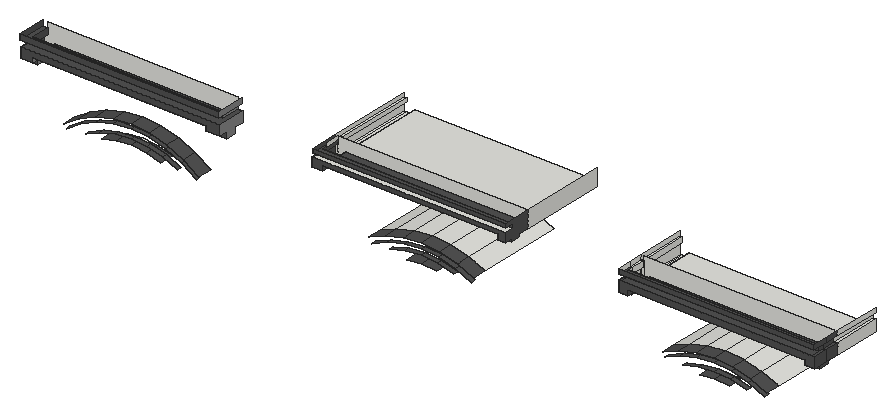
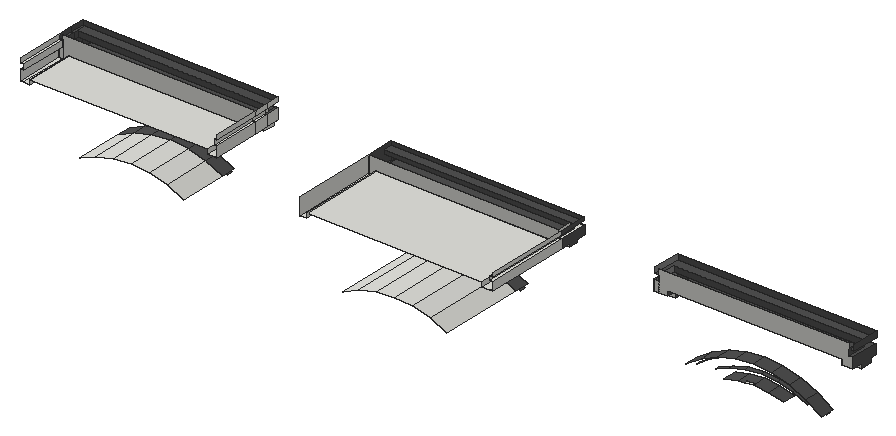
# SketchUp Ruby script. Lengths in inches.
U = 1.inch
M = Sketchup.active_model
def pt(a) = Geom::Point3d.new(a.map { |v| v * U })
def face(e, loops, mat)
  f = e.add_face(loops[0].map { |a| pt(a) })
  loops[1..].each { |l| e.add_face(l.map { |a| pt(a) }).erase! }
  f.material = f.back_material = mat if mat
  f
end
# faces: each face lists its corners as indices into pts; further lists are holes
def faces(e, pts, list, mat = nil) = list.each { |f| face(e, (f[0].is_a?(Array) ? f : [f]).map { |l| l.map { |i| pts[i] } }, mat) }
# xy, xz, yz: faces in a plane at the given z, y or x. An outline is a flat list of corners, or four numbers for a rectangle; further outlines are holes
def ring(l) = l.size == 4 ? [[l[0], l[1]], [l[2], l[1]], [l[2], l[3]], [l[0], l[3]]] : l.each_slice(2).to_a
def flat(e, list, mat, &to3) = list.each { |f| face(e, (f[0].is_a?(Array) ? f : [f]).map { |l| ring(l).map { |u, v| to3.(u, v) } }, mat) }
def xy(e, z, list, mat = nil) = flat(e, list, mat) { |x, y| [x, y, z] }
def xz(e, y, list, mat = nil) = flat(e, list, mat) { |x, z| [x, y, z] }
def yz(e, x, list, mat = nil) = flat(e, list, mat) { |y, z| [x, y, z] }
def lines(e, pts, list) = list.each { |a, b| e.add_line(pt(pts[a]), pt(pts[b])) }
# prism: a flat outline (further loops are holes) pulled along v
def prism(e, loops, v, mat = nil)
  f = face(e, loops, mat); d = Geom::Vector3d.new(v.map { |x| x * U })
  f.pushpull(f.normal.samedirection?(d) ? d.length : -d.length)
end
def box(e, o, s, mat = nil) = prism(e, [[o, [o[0] + s[0], o[1], o[2]], [o[0] + s[0], o[1] + s[1], o[2]], [o[0], o[1] + s[1], o[2]]]], [0, 0, s[2]], mat)
def at(x, y, z, deg = 0) = Geom::Transformation.translation(pt([x, y, z])) * Geom::Transformation.rotation(ORIGIN, Z_AXIS, deg.degrees)
def axes(o, x, y, z) = Geom::Transformation.new([*x, 0, *y, 0, *z, 0, *pt(o).to_a, 1])
def part(name) = M.definitions.add(name)
# library, detail: a bought-in or finely detailed component or shape, given as its bounding box
def library(name, o, s) = part(name).tap { |d| box(d.entities, o, s) }
def detail(e, o, s) = box(e.add_group.entities, o, s)
def put(e, d, t, mat = nil) = e.add_instance(d, t).tap { |i| i.material = mat if mat }
def group(e, t, mat = nil) = e.add_group.tap { |g| g.transformation = t; g.material = mat if mat }.entities
root = M.entities
M.materials.add("[0133_Gray]").color = [135, 135, 135]
M.materials.add("[0135_DarkGray]").color = [81, 81, 81]
xy(root,319.41,[[171.09,37.19,179.82,43.47]],"[0135_DarkGray]")
xy(root,320.41,[[53.26,35.48,60.625,42.85]],"[0133_Gray]")
xy(root,322.03,[[551.95,35.67,558.14,41.86]],"[0135_DarkGray]")
xy(root,322.22,[[433.26,35.43,438.96,42.62]],"[0135_DarkGray]")
xy(root,323.16,[[53.26,31.6875,60.625,35.48],[53.26,42.85,60.625,49.6875]],"[0133_Gray]")
xy(root,323.16,[[171.09,31.6875,179.82,37.19],[171.09,43.47,179.82,49.6875]],"[0135_DarkGray]")
xy(root,323.47,[[433.26,35.43,434.7,40.6875],[434.7,35.43,438.96,40.6875],[551.95,35.67,556.01,40.6875],[556.01,35.67,558.14,40.6875],[433.26,40.6875,434.7,42.62],
  [434.7,40.6875,438.96,42.62],[551.95,40.6875,556.01,41.86],[556.01,40.6875,558.14,41.86],[433.26,49.6875,434.7,80.4375],[434.7,49.6875,438.96,80.4375],
  [551.95,49.6875,556.01,80.4375],[556.01,49.6875,558.14,80.4375]])
xy(root,323.47,[[433.26,31.6875,434.7,35.43],[434.7,31.6875,438.96,35.43],[551.95,31.6875,556.01,35.67],[556.01,31.6875,558.14,35.67],[551.95,41.86,556.01,49.6875],
  [556.01,41.86,558.14,49.6875],[433.26,42.62,434.7,49.6875],[434.7,42.62,438.96,49.6875]],"[0135_DarkGray]")
xy(root,324.72,[[356.5625,36.9,361.32,42.55]],"[0135_DarkGray]")
xy(root,324.91,[[238.45,37.86,245.25,43.34]],"[0135_DarkGray]")
xy(root,326.16,[[60.625,31.6875,171.09,49.6875]],"[0135_DarkGray]")
xy(root,326.47,[[238.45,49.6875,240.45,104.375],[240.45,49.6875,245.25,104.375],[356.5625,49.6875,361.32,104.375],[438.96,49.6875,551.95,80.4375]])
xy(root,326.47,[[238.45,31.6875,245.25,37.86],[356.5625,31.6875,361.32,36.9],[438.96,31.6875,551.95,49.6875],[356.5625,42.55,361.32,49.6875],[238.45,43.34,245.25,49.6875]],"[0135_DarkGray]")
xy(root,329.47,[[245.25,49.6875,356.5625,104.375]])
xy(root,329.47,[[245.25,31.6875,356.5625,49.6875]],"[0135_DarkGray]")
xy(root,329.79,[[53.26,31.6875,179.82,31.6875,179.82,49.6875,176.89,49.6875,176.89,37.6875,55.95,37.6875,55.95,49.6875,53.26,49.6875]],"[0135_DarkGray]")
xy(root,330.36,[[433.26,40.6875,434.7,49.6875],[433.26,49.6875,434.7,80.4375],[556.01,49.6875,558.14,80.4375]])
xy(root,330.36,[[433.26,31.6875,434.7,40.6875],[434.7,31.6875,556.01,37.6875],[556.01,31.6875,558.14,40.6875],[556.01,40.6875,558.14,49.6875]],"[0135_DarkGray]")
xy(root,332.04,[[238.45,31.6875,361.32,31.6875,361.32,37.6875,240.45,37.6875,240.45,49.6875,238.45,49.6875],[238.45,49.6875,240.45,104.375]])
xy(root,333.42,[[52.82,31.6875,52.82,49.6875,55.95,49.6875,55.95,37.6875,176.89,37.6875,176.89,49.6875,179.26,49.6875,179.26,31.6875]],"[0135_DarkGray]")
xy(root,334.01,[[433.14,40.6875,434.7,49.6875],[433.14,49.6875,434.7,80.4375],[556.01,49.6875,557.64,80.4375]])
xy(root,334.01,[[433.14,31.6875,434.7,40.6875],[434.7,31.6875,556.01,37.6875],[556.01,31.6875,557.64,40.6875],[556.01,40.6875,557.64,49.6875]],"[0135_DarkGray]")
xy(root,334.61,[[238.64,49.6875,240.45,104.375]])
xy(root,334.61,[[238.64,31.6875,238.64,49.6875,240.45,49.6875,240.45,37.6875,361.32,37.6875,361.32,31.6875]],"[0135_DarkGray]")
xz(root,31.6875,[[53.26,323.16,60.625,323.16,60.625,326.16,171.09,326.16,171.09,323.16,179.82,323.16,179.82,329.79,53.26,329.79],[433.26,323.47,438.96,323.47,438.96,326.47,551.95,326.47,551.95,323.47,558.14,323.47,558.14,330.36,433.26,330.36],[238.45,326.47,245.25,326.47,245.25,329.47,356.5625,329.47,356.5625,326.47,361.32,326.47,361.32,332.04,238.45,332.04],[52.82,333.42,179.26,336.85],[433.14,334.01,557.64,336.85],
  [238.64,334.61,361.32,336.85]],"[0135_DarkGray]")
xz(root,35.43,[[433.26,322.22,438.96,323.47]],"[0135_DarkGray]")
xz(root,35.48,[[53.26,320.41,60.625,323.16]],"[0135_DarkGray]")
xz(root,35.67,[[551.95,322.03,558.14,323.47]],"[0135_DarkGray]")
xz(root,36.9,[[356.5625,324.72,361.32,326.47]],"[0135_DarkGray]")
xz(root,37.19,[[171.09,319.41,179.82,323.16]],"[0135_DarkGray]")
xz(root,37.6875,[[55.95,329.79,176.89,333.42],[434.7,330.36,556.01,334.01],[240.45,332.04,361.32,334.61]],"[0135_DarkGray]")
xz(root,37.86,[[238.45,324.91,245.25,326.47]],"[0135_DarkGray]")
xz(root,41.86,[[551.95,322.03,558.14,323.47]])
xz(root,42.55,[[356.5625,324.72,361.32,326.47]])
xz(root,42.62,[[433.26,322.22,438.96,323.47]])
xz(root,42.85,[[53.26,320.41,60.625,323.16]])
xz(root,43.34,[[238.45,324.91,245.25,326.47]])
xz(root,43.47,[[171.09,319.41,179.82,323.16]])
xz(root,49.6875,[[53.26,323.16,60.625,323.16,60.625,326.16,171.09,326.16,171.09,323.16,176.89,323.16,176.89,336.85,55.95,336.85,55.95,329.79,53.26,329.79],[176.89,323.16,179.82,329.79],[433.26,323.47,434.7,330.36],[434.7,323.47,434.7,336.85,556.01,336.85,556.01,323.47,551.95,323.47,551.95,326.47,438.96,326.47,438.96,323.47],[556.01,323.47,558.14,330.36],
  [238.45,326.47,240.45,332.04],[240.45,326.47,245.25,326.47,245.25,329.47,356.5625,329.47,356.5625,326.47,361.32,326.47,361.32,336.85,240.45,336.85]])
yz(root,52.82,[[31.6875,333.42,49.6875,336.85]],"[0135_DarkGray]")
yz(root,53.26,[[35.48,320.41,35.48,323.16,31.6875,323.16,31.6875,329.79,49.6875,329.79,49.6875,323.16,42.85,323.16,42.85,320.41]],"[0135_DarkGray]")
yz(root,55.95,[[37.6875,329.79,49.6875,333.42]],"[0135_DarkGray]")
yz(root,60.625,[[35.48,320.41,42.85,320.41,42.85,323.16,49.6875,323.16,49.6875,326.16,31.6875,326.16,31.6875,323.16,35.48,323.16]],"[0133_Gray]")
yz(root,171.09,[[37.19,319.41,37.19,323.16,31.6875,323.16,31.6875,326.16,49.6875,326.16,49.6875,323.16,43.47,323.16,43.47,319.41]],"[0135_DarkGray]")
yz(root,176.89,[[37.6875,329.79,49.6875,333.42]],"[0133_Gray]")
yz(root,179.26,[[31.6875,333.42,49.6875,336.85]],"[0133_Gray]")
yz(root,179.82,[[37.19,319.41,43.47,319.41,43.47,323.16,49.6875,323.16,49.6875,329.79,31.6875,329.79,31.6875,323.16,37.19,323.16]],"[0133_Gray]")
yz(root,238.45,[[49.6875,326.47,104.375,332.04]])
yz(root,238.45,[[37.86,324.91,37.86,326.47,31.6875,326.47,31.6875,332.04,49.6875,332.04,49.6875,326.47,43.34,326.47,43.34,324.91]],"[0135_DarkGray]")
yz(root,238.64,[[49.6875,334.61,104.375,336.85]])
yz(root,238.64,[[31.6875,334.61,49.6875,336.85]],"[0135_DarkGray]")
yz(root,240.45,[[49.6875,332.04,104.375,334.61],[40.6875,334.61,49.6875,336.85]])
yz(root,240.45,[[37.6875,332.04,49.6875,334.61]],"[0135_DarkGray]")
yz(root,245.25,[[49.6875,326.47,104.375,329.47]])
yz(root,245.25,[[37.86,324.91,43.34,324.91,43.34,326.47,49.6875,326.47,49.6875,329.47,31.6875,329.47,31.6875,326.47,37.86,326.47]],"[0135_DarkGray]")
yz(root,356.5625,[[49.6875,326.47,104.375,329.47]])
yz(root,356.5625,[[36.9,324.72,36.9,326.47,31.6875,326.47,31.6875,329.47,49.6875,329.47,49.6875,326.47,42.55,326.47,42.55,324.72]],"[0135_DarkGray]")
yz(root,361.32,[[49.6875,326.47,104.375,336.85]])
yz(root,361.32,[[36.9,324.72,42.55,324.72,42.55,326.47,49.6875,326.47,49.6875,336.85,31.6875,336.85,31.6875,334.61,37.6875,334.61,37.6875,332.04,31.6875,332.04,31.6875,326.47,36.9,326.47]],"[0135_DarkGray]")
yz(root,433.14,[[31.6875,334.01,40.6875,336.85],[40.6875,334.01,49.6875,336.85],[49.6875,334.01,80.4375,336.85]])
yz(root,433.26,[[35.43,322.22,42.62,323.47],[31.6875,323.47,40.6875,330.36],[40.6875,323.47,49.6875,330.36],[49.6875,323.47,80.4375,330.36]])
yz(root,434.7,[[37.6875,330.36,40.6875,334.01],[40.6875,330.36,49.6875,334.01],[49.6875,330.36,80.4375,334.01]])
yz(root,438.96,[[49.6875,323.47,80.4375,326.47]])
yz(root,438.96,[[35.43,322.22,42.62,323.47],[31.6875,323.47,40.6875,326.47],[40.6875,323.47,49.6875,326.47]],"[0135_DarkGray]")
yz(root,551.95,[[35.67,322.03,41.86,323.47],[31.6875,323.47,40.6875,326.47],[40.6875,323.47,49.6875,326.47],[49.6875,323.47,80.4375,326.47]])
yz(root,556.01,[[49.6875,330.36,80.4375,334.01]])
yz(root,556.01,[[37.6875,330.36,40.6875,334.01],[40.6875,330.36,49.6875,334.01]],"[0135_DarkGray]")
yz(root,557.64,[[49.6875,334.01,80.4375,336.85]])
yz(root,557.64,[[31.6875,334.01,40.6875,336.85],[40.6875,334.01,49.6875,336.85]],"[0135_DarkGray]")
yz(root,558.14,[[49.6875,323.47,80.4375,330.36]])
yz(root,558.14,[[35.67,322.03,41.86,323.47],[31.6875,323.47,40.6875,330.36],[40.6875,323.47,49.6875,330.36]],"[0135_DarkGray]")
p = [[75.01,43.6875,286.86],[84.29,43.6875,292.97],[84.29,40.6875,292.97],[75.01,40.6875,286.86],[148.3,43.6875,292.97],[157.58,43.6875,286.86],
  [157.58,40.6875,286.86],[148.3,40.6875,292.97],[310.32,49.6875,288.18],[311.64,49.6875,287.84],[311.64,47.6875,287.84],[310.32,47.6875,288.18],
  [96.3,43.6875,292.1],[87,43.6875,287.99],[87,40.6875,287.99],[96.3,40.6875,292.1],[145.58,43.6875,287.99],[136.28,43.6875,292.1],
  [136.28,40.6875,292.1],[145.58,40.6875,287.99],[291.27,49.6875,288.18],[300.79,49.6875,288.97],[300.79,40.6875,288.97],[291.27,40.6875,288.18],
  [305.64,49.6875,288.57],[305.64,47.6875,288.57],[310.32,40.6875,288.18],[477.77,49.6875,288.18],[483.7,49.6875,288.67],[483.7,47.6875,288.67],
  [487.29,47.6875,288.97],[487.29,40.6875,288.97],[477.77,40.6875,288.18],[489.7,47.6875,288.77],[489.7,49.6875,288.77],[496.82,49.6875,288.18],
  [496.82,40.6875,288.18],[97.5,49.6875,288.63],[106.77,49.6875,290.99],[106.77,40.6875,290.99],[97.5,40.6875,288.63],[125.82,49.6875,290.99],
  [135.08,49.6875,288.63],[135.08,40.6875,288.63],[125.82,40.6875,290.99],[487.29,49.6875,288.97],[83,49.6875,295.34],[73.34,49.6875,288.98],
  [73.34,40.6875,288.98],[83,40.6875,295.34],[159.24,49.6875,288.98],[149.59,49.6875,295.34],[149.59,40.6875,295.34],[159.24,40.6875,288.98],
  [269.16,43.6875,289.48],[279.2,43.6875,293.92],[279.2,40.6875,293.92],[269.16,40.6875,289.48],[322.38,43.6875,293.92],[332.43,43.6875,289.48],
  [332.43,40.6875,289.48],[322.38,40.6875,293.92],[477.06,43.6875,292.35],[467.12,43.6875,289.82],[467.12,40.6875,289.82],[477.06,40.6875,292.35],
  [507.46,43.6875,289.82],[497.52,43.6875,292.35],[497.52,40.6875,292.35],[507.46,40.6875,289.82],[455.29,43.6875,290.15],[465.45,43.6875,294.64],
  [465.45,40.6875,294.64],[455.29,40.6875,290.15],[509.13,43.6875,294.64],[519.29,43.6875,290.15],[519.29,40.6875,290.15],[509.13,40.6875,294.64],
  [290.44,43.6875,293.07],[280.38,43.6875,290.5],[280.38,40.6875,290.5],[290.44,40.6875,293.07],[321.2,43.6875,290.5],[311.14,43.6875,293.07],
  [311.14,40.6875,293.07],[321.2,40.6875,290.5],[116.29,49.6875,291.78],[116.29,47.6875,291.78],[116.29,40.6875,291.78],[122.29,47.6875,291.28],
  [122.29,49.6875,291.28],[106.16,43.6875,294.61],[106.16,40.6875,294.61],[126.42,43.6875,294.61],[126.42,40.6875,294.61],[487.29,43.6875,293.21],
  [487.29,40.6875,293.21],[278.07,49.6875,297.2],[267.5,49.6875,292.53],[267.5,40.6875,292.53],[278.07,40.6875,297.2],[334.09,49.6875,292.53],
  [323.51,49.6875,297.2],[323.51,40.6875,297.2],[334.09,40.6875,292.53],[454,49.6875,292.53],[464.57,49.6875,297.2],[464.57,40.6875,297.2],
  [454,40.6875,292.53],[510.01,49.6875,297.2],[520.59,49.6875,292.53],[520.59,40.6875,292.53],[510.01,40.6875,297.2],[267.5,104.375,292.53],
  [278.07,104.375,297.2],[323.51,104.375,297.2],[334.09,104.375,292.53],[454,80.4375,292.53],[464.57,80.4375,297.2],[510.01,80.4375,297.2],
  [520.59,80.4375,292.53],[94.45,43.6875,297.46],[94.45,40.6875,297.46],[138.13,43.6875,297.46],[138.13,40.6875,297.46],[300.79,43.6875,293.93],
  [300.79,40.6875,293.93],[289.85,43.6875,296.64],[289.85,40.6875,296.64],[311.74,43.6875,296.64],[311.74,40.6875,296.64],[116.29,43.6875,295.46],
  [116.29,40.6875,295.46],[476.22,43.6875,297.38],[476.22,40.6875,297.38],[498.36,43.6875,297.38],[498.36,40.6875,297.38],[93.57,49.6875,300.01],
  [93.57,40.6875,300.01],[139.01,49.6875,300.01],[139.01,40.6875,300.01],[300.79,43.6875,297.55],[300.79,40.6875,297.55],[289.27,49.6875,300.05],
  [289.27,40.6875,300.05],[312.3125,49.6875,300.05],[312.3125,40.6875,300.05],[475.77,49.6875,300.05],[475.77,40.6875,300.05],[498.8125,49.6875,300.05],
  [498.8125,40.6875,300.05],[289.27,104.375,300.05],[312.3125,104.375,300.05],[475.77,80.4375,300.05],[498.8125,80.4375,300.05],[487.29,43.6875,298.31],
  [487.29,40.6875,298.31],[105.22,43.6875,300.21],[105.22,40.6875,300.21],[127.36,43.6875,300.21],[127.36,40.6875,300.21],[104.77,49.6875,302.86],
  [104.77,40.6875,302.86],[127.8125,49.6875,302.86],[127.8125,40.6875,302.86],[300.79,49.6875,301.01],[300.79,40.6875,301.01],[487.29,49.6875,301.01],
  [487.29,40.6875,301.01],[300.79,104.375,301.01],[487.29,80.4375,301.01],[116.29,43.6875,301.13],[116.29,40.6875,301.13],[116.29,49.6875,303.82],
  [116.29,40.6875,303.82],[176.89,37.6875,329.79],[176.89,37.6875,326.16],[240.45,37.6875,334.61],[240.45,37.6875,336.85],[240.45,37.6875,329.47],
  [240.45,37.6875,332.04],[434.7,37.6875,334.01],[434.7,37.6875,336.85],[556.01,37.6875,330.36],[556.01,37.6875,326.47],[434.7,37.6875,326.47],
  [434.7,37.6875,330.36],[122.29,49.6875,291.39]]
faces(root,p,[[0,1,2,3],[4,5,6,7],[12,13,14,15],[16,17,18,19],[20,21,22,23],[21,24,25,11,26,22],[27,28,29,30,31,32],[31,30,33,34,35,36],
  [37,38,39,40],[41,42,43,44],[46,47,48,49],[50,51,52,53],[54,55,56,57],[58,59,60,61],[62,63,64,65],[66,67,68,69],
  [70,71,72,73],[74,75,76,77],[78,79,80,81],[82,83,84,85],[38,86,87,88,39],[88,87,89,90,41,44],[91,12,15,92],[17,93,94,18],
  [95,62,65,96],[67,95,96,68],[97,98,99,100],[101,102,103,104],[105,106,107,108],[109,110,111,112],[1,121,122,2],[123,4,7,124],
  [125,78,81,126],[83,125,126,84],[55,127,128,56],[129,58,61,130],[131,91,92,132],[93,131,132,94],[71,133,134,72],[135,74,77,136],
  [137,46,49,138],[51,139,140,52],[127,141,142,128],[141,129,130,142],[143,97,100,144],[102,145,146,103],[106,147,148,107],[149,109,112,150],
  [133,155,156,134],[155,135,136,156],[121,157,158,122],[159,123,124,160],[161,137,138,162],[139,163,164,140],[165,143,144,166],[145,165,166,146],
  [147,167,168,148],[167,149,150,168],[157,171,172,158],[171,159,160,172],[173,161,162,174],[163,173,174,164]],"[0135_DarkGray]")
faces(root,p,[[8,9,10,11],[24,8,11,25],[28,45,30,29],[45,34,33,30],[86,90,89,87],[97,98,113,114],[101,102,115,116],[106,105,117,118],
  [110,109,119,120],[143,97,114,151],[102,145,152,115],[147,106,118,153],[109,149,154,119],[165,143,151,169],[145,165,169,152],[167,147,153,170],
  [149,167,170,154]])
lines(root,p,[[175,176],[177,178],[179,180],[181,182],[183,184],[185,186],[90,187]])
